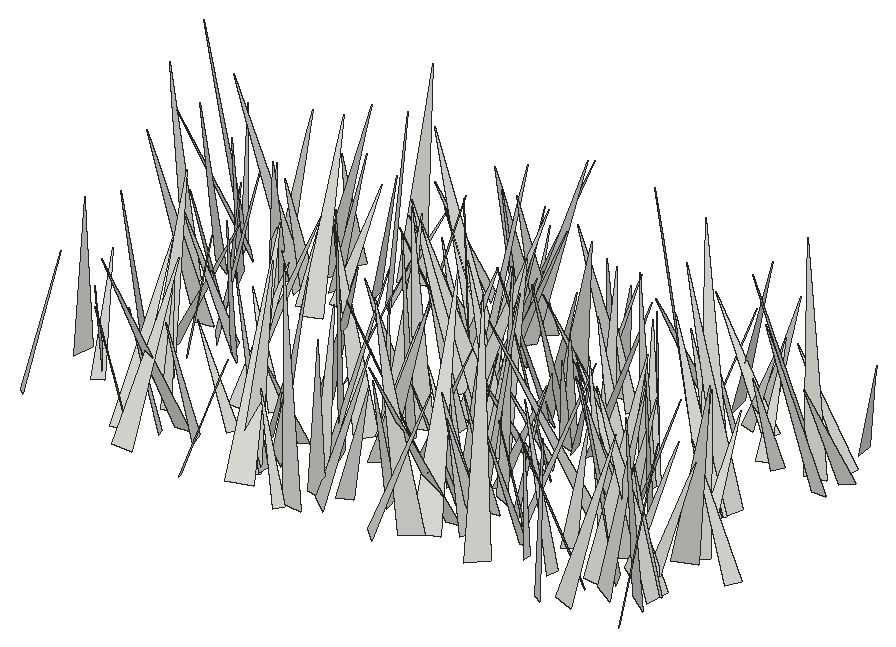
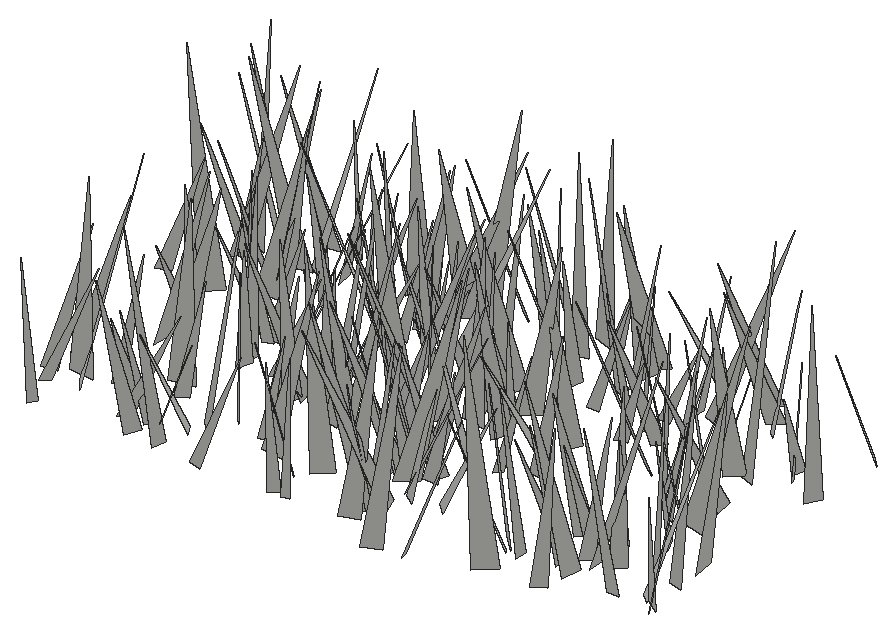
# SketchUp Ruby script. Lengths in inches.
U = 1.inch
M = Sketchup.active_model
def pt(a) = Geom::Point3d.new(a.map { |v| v * U })
def face(e, loops, mat)
  f = e.add_face(loops[0].map { |a| pt(a) })
  loops[1..].each { |l| e.add_face(l.map { |a| pt(a) }).erase! }
  f.material = f.back_material = mat if mat
  f
end
# faces: each face lists its corners as indices into pts; further lists are holes
def faces(e, pts, list, mat = nil) = list.each { |f| face(e, (f[0].is_a?(Array) ? f : [f]).map { |l| l.map { |i| pts[i] } }, mat) }
# xy, xz, yz: faces in a plane at the given z, y or x. An outline is a flat list of corners, or four numbers for a rectangle; further outlines are holes
def ring(l) = l.size == 4 ? [[l[0], l[1]], [l[2], l[1]], [l[2], l[3]], [l[0], l[3]]] : l.each_slice(2).to_a
def flat(e, list, mat, &to3) = list.each { |f| face(e, (f[0].is_a?(Array) ? f : [f]).map { |l| ring(l).map { |u, v| to3.(u, v) } }, mat) }
def xy(e, z, list, mat = nil) = flat(e, list, mat) { |x, y| [x, y, z] }
def xz(e, y, list, mat = nil) = flat(e, list, mat) { |x, z| [x, y, z] }
def yz(e, x, list, mat = nil) = flat(e, list, mat) { |y, z| [x, y, z] }
def lines(e, pts, list) = list.each { |a, b| e.add_line(pt(pts[a]), pt(pts[b])) }
# prism: a flat outline (further loops are holes) pulled along v
def prism(e, loops, v, mat = nil)
  f = face(e, loops, mat); d = Geom::Vector3d.new(v.map { |x| x * U })
  f.pushpull(f.normal.samedirection?(d) ? d.length : -d.length)
end
def box(e, o, s, mat = nil) = prism(e, [[o, [o[0] + s[0], o[1], o[2]], [o[0] + s[0], o[1] + s[1], o[2]], [o[0], o[1] + s[1], o[2]]]], [0, 0, s[2]], mat)
def at(x, y, z, deg = 0) = Geom::Transformation.translation(pt([x, y, z])) * Geom::Transformation.rotation(ORIGIN, Z_AXIS, deg.degrees)
def axes(o, x, y, z) = Geom::Transformation.new([*x, 0, *y, 0, *z, 0, *pt(o).to_a, 1])
def part(name) = M.definitions.add(name)
# library, detail: a bought-in or finely detailed component or shape, given as its bounding box
def library(name, o, s) = part(name).tap { |d| box(d.entities, o, s) }
def detail(e, o, s) = box(e.add_group.entities, o, s)
def put(e, d, t, mat = nil) = e.add_instance(d, t).tap { |i| i.material = mat if mat }
def group(e, t, mat = nil) = e.add_group.tap { |g| g.transformation = t; g.material = mat if mat }.entities
root = M.entities
c1 = part("fur_instance\#9")
p = [[0.8125,0,1.79],[0.67,-0.02,1.48],[0,-0.11,0],[0,0.11,0]]
faces(c1.entities,p,[[0,1,2,3]])
put(root,c1,axes([469.1875,380.91,-21.66],[3.38601,2.0667,0.33408],[1.88033,-3.28152,1.24252],[-0.92044,0.89903,3.76728]))
put(root,c1,axes([476.36,381.6,-21.66],[-0.98772,3.5916,0.11089],[3.35733,0.88143,1.35606],[-1.28071,-0.45933,3.46934]))
put(root,c1,axes([476.99,382.05,-21.66],[1.25442,7.48082,2.76942],[7.81491,-1.71475,1.09211],[-1.59984,-2.51056,7.50623]))
put(root,c1,axes([477.25,384.18,-21.66],[0.11264,-6.37998,1.60761],[-6.5012,0.13924,1.0081],[1.01142,1.60553,6.30084]))
put(root,c1,axes([462.07,384.52,-21.66],[-3.11173,-3.4795,0.92655],[-3.33661,3.24675,0.98692],[1.3537,0.0043,4.56244]))
put(root,c1,axes([482.78,382.4,-21.66],[3.70587,4.25797,0.60198],[4.28884,-3.60158,-0.92773],[0.31394,-1.06043,5.56805]))
put(root,c1,axes([495.72,382.58,-21.66],[2.53366,4.26731,1.78001],[4.34271,-2.89305,0.75426],[-1.5872,-1.10369,4.90515]))
put(root,c1,axes([496.5,385.9375,-21.66],[-4.09518,-5.32392,0.52178],[-5.17841,4.11019,1.29512],[1.34181,-0.38619,6.5907]))
put(root,c1,axes([465.73,385.54,-21.66],[-1.54524,-6.7658,0.51217],[-6.71547,1.44992,-1.10738],[-0.96994,0.74015,6.85109]))
put(root,c1,axes([464.27,381.45,-21.66],[-1.14169,6.19263,0.48775],[6.13199,1.20279,-0.91762],[0.99261,-0.30768,6.22978]))
put(root,c1,axes([478.04,383.45,-21.66],[3.54049,4.95211,1.34575],[5.12044,-3.30078,-1.32493],[0.33991,-1.85767,5.94164]))
put(root,c1,axes([467.2,385.05,-21.66],[-4.25466,-1.2014,1.34721],[-0.93808,4.41863,0.97784],[1.54219,-0.62673,4.31153]))
put(root,c1,axes([484.75,383.99,-21.66],[1.79805,-6.87497,3.712],[-7.43664,-2.674,-1.35027],[-2.39594,3.14033,6.97674]))
put(root,c1,axes([497.25,383.15,-21.66],[1.23681,5.98503,1.54047],[6.1022,-0.934,-1.27052],[0.97821,-1.7408,5.97797]))
put(root,c1,axes([478.81,384.96,-21.66],[3.21186,-3.52218,0.8528],[-3.62385,-3.13,0.72104],[-0.02677,1.11644,4.71189]))
put(root,c1,axes([464.93,384.375,-21.66],[-3.69691,-1.68274,0.52652],[-1.75981,3.59718,-0.85985],[0.10916,1.00233,3.96981]))
put(root,c1,axes([485.88,386.71,-21.66],[-1.10699,-6.38687,0.31821],[-6.26084,1.01671,-1.37367],[-1.30201,0.54128,6.33487]))
put(root,c1,axes([501.52,383.35,-21.66],[-4.45958,-2.36263,3.46386],[-3.3219,5.07642,-0.81428],[2.55838,2.47306,4.98064]))
put(root,c1,axes([500.88,385.89,-21.66],[-3.13728,-6.42445,2.27927],[-6.51063,3.56742,1.09378],[2.01998,1.52023,7.06539]))
put(root,c1,axes([455.16,383.0625,-21.66],[3.04107,3.48011,0.59696],[3.3547,-3.09349,0.94446],[-1.10161,0.1866,4.52408]))
put(root,c1,axes([472.42,383.6875,-21.66],[-5.70861,3.53079,2.01517],[3.32922,6.05385,-1.17592],[2.33318,0.00055,6.60847]))
put(root,c1,axes([481.35,386.33,-21.66],[4.6906,-0.13116,1.94102],[0.35682,-4.92253,-1.19491],[-1.91244,-1.24013,4.53774]))
put(root,c1,axes([487.46,386.14,-21.66],[3.16597,-2.82128,1.36449],[-2.73379,-3.43456,-0.75836],[-1.53229,0.2984,4.17228]))
put(root,c1,axes([487.93,386.76,-21.66],[2.45481,-4.16097,0.8917],[-4.06011,-2.59844,-0.9479],[-1.27449,0.26329,4.73722]))
put(root,c1,axes([472.73,384.6,-21.66],[-6.0397,-1.24718,1.08354],[-1.47294,5.92489,-1.39057],[0.74831,1.59618,6.00831]))
put(root,c1,axes([462.74,383.22,-21.66],[-1.71935,6.00909,0.23442],[5.94835,1.73522,-0.85232],[0.8839,0.01135,6.19184]))
put(root,c1,axes([472.59,382.47,-21.66],[-4.41357,6.91206,0.00056],[6.86097,4.38103,-0.99489],[0.83882,0.53496,8.14041]))
put(root,c1,axes([472.5,386.22,-21.66],[-2.78435,-5.66723,3.39056],[-5.97834,3.72634,1.319],[2.80584,2.3158,6.17497]))
put(root,c1,axes([486.87,387.5,-21.66],[-3.71631,2.59474,2.95715],[3.6126,3.86147,1.15179],[1.55775,-2.76492,4.38373]))
put(root,c1,axes([489.99,383.9,-21.66],[-7.18499,4.19207,1.05141],[4.04317,7.24035,-1.23823],[1.52698,0.55406,8.22584]))
put(root,c1,axes([498.52,385.55,-21.66],[3.30058,6.51639,2.13105],[6.85171,-3.21879,-0.76942],[-0.24255,-2.25268,7.26396]))
put(root,c1,axes([494.46,385.62,-21.66],[-5.51822,-0.21879,0.79161],[-0.32668,5.51842,-0.75206],[0.75352,0.79022,5.4711]))
put(root,c1,axes([501.37,387.21,-21.66],[-7.04891,1.70289,1.4017],[1.92518,7.04086,1.12767],[1.07622,-1.44158,7.16347]))
put(root,c1,axes([492.04,386.14,-21.66],[-3.53666,-0.44387,1.07965],[-0.6619,3.59984,-0.68824],[0.96154,0.84544,3.49732]))
put(root,c1,axes([490.95,387.22,-21.66],[-2.05485,-3.90462,0.97999],[-3.96047,1.76344,-1.27819],[-0.72186,1.43981,4.22312]))
put(root,c1,axes([486.05,387.56,-21.66],[-2.14589,-4.13922,0.79032],[-4.13009,1.88974,-1.31675],[-0.83673,1.28775,4.4726]))
put(root,c1,axes([457.51,388.1,-21.66],[3.15596,1.30372,1.61225],[1.82364,-3.14251,-1.02861],[-0.98659,-1.6383,3.25603]))
put(root,c1,axes([470.65,387.78,-21.66],[3.7872,-0.0255,0.26622],[0.02172,-3.73751,-0.66706],[-0.26655,-0.66693,3.72808]))
put(root,c1,axes([483.1,388.82,-21.66],[-4.92734,-5.46841,0.2776],[-5.45988,4.87887,-0.80338],[-0.41255,0.74316,7.31688]))
put(root,c1,axes([501.12,387.38,-21.66],[-0.94166,-4.10224,1.61468],[-4.38512,0.70145,-0.77524],[-0.45421,1.73259,4.13692]))
put(root,c1,axes([498.1,387.43,-21.66],[-6.28358,-3.49392,1.76213],[-3.72095,6.36668,-0.64478],[1.21124,1.43309,7.16066]))
put(root,c1,axes([472.57,388.79,-21.66],[0.53786,-3.60504,0.14249],[-3.55289,-0.5543,-0.6129],[-0.62738,0.04841,3.59304]))
put(root,c1,axes([485.4375,384.55,-21.66],[-4.43994,6.98412,0.3729],[6.94517,4.45476,-0.74146],[0.82561,0.08476,8.24265]))
put(root,c1,axes([468.29,387.21,-21.66],[-1.80359,3.13263,0.44398],[3.00697,1.53819,1.36218],[-0.98418,-1.04117,3.34825]))
put(root,c1,axes([497.26,386.28,-21.66],[0.16612,7.76506,1.97129],[7.95416,0.07536,-0.96713],[0.95574,-1.97685,7.70638]))
put(root,c1,axes([463.5,386.73,-21.66],[0.00503,4.167,0.7042],[4.17874,-0.11,0.62111],[-0.63075,-0.69557,4.12045]))
put(root,c1,axes([468.43,389.13,-21.66],[4.23217,0.79223,1.75299],[1.35483,-4.23497,-1.35698],[-1.36567,-1.74623,4.08626]))
put(root,c1,axes([459.77,389.8,-21.66],[-3.5221,-6.63629,1.77015],[-6.5539,3.84233,1.36448],[2.0543,0.8804,7.38808]))
put(root,c1,axes([489.56,389.01,-21.66],[-3.13954,-2.86345,1.03549],[-2.74612,3.30524,0.81394],[1.31545,0.06589,4.17056]))
put(root,c1,axes([500.37,387.43,-21.66],[0.61438,4.77457,1.24038],[4.786,-0.27399,-1.3159],[1.1955,-1.35681,4.63059]))
put(root,c1,axes([475.31,387.11,-21.66],[-4.49774,2.41965,1.22715],[2.26445,4.65664,-0.88215],[1.49428,0.22634,5.03052]))
put(root,c1,axes([454.97,389.32,-21.66],[5.79339,-2.08626,1.56673],[-1.97661,-6.00002,-0.68061],[-1.70297,-0.13319,6.11985]))
put(root,c1,axes([496.99,390.07,-21.66],[1.49882,-6.76146,1.59023],[-6.75855,-1.79498,-1.262],[-1.60255,1.24632,6.80963]))
put(root,c1,axes([487.15,389.16,-21.66],[-0.77658,-4.10323,1.17838],[-4.23531,0.59015,-0.73621],[-0.53592,1.28194,4.11067]))
put(root,c1,axes([457.85,387.13,-21.66],[-3.33951,2.40161,0.05247],[2.31618,3.24301,-1.02031],[0.63702,0.79874,3.98485]))
put(root,c1,axes([497.44,387.4375,-21.66],[-6.80477,1.06742,0.77743],[0.9228,6.76292,-1.20833],[0.94457,1.0827,6.78117]))
put(root,c1,axes([493.25,388.74,-21.66],[3.51253,-2.51047,1.78394],[-2.89575,-3.6135,0.61652],[-1.0486,1.56939,4.2732]))
put(root,c1,axes([482.89,390.39,-21.66],[3.48904,-1.79502,0.75996],[-1.60226,-3.52839,-0.97792],[-1.11014,-0.54905,3.7999]))
put(root,c1,axes([488.62,389.24,-21.66],[2.69077,3.3772,1.27263],[3.60609,-2.57991,-0.77814],[-0.14558,-1.48455,4.24737]))
put(root,c1,axes([498.06,388.5,-21.66],[2.30047,4.4169,0.81433],[4.47004,-2.16262,-0.89782],[0.43686,-1.13065,4.89848]))
put(root,c1,axes([487.16,387.67,-21.66],[4.31579,6.0344,1.65644],[5.97789,-4.5707,1.07586],[-1.85004,-0.69181,7.34048]))
put(root,c1,axes([475.23,387.58,-21.66],[4.30738,5.01035,0.65824],[4.94004,-4.35705,0.83813],[-1.06435,0.05398,6.55397]))
put(root,c1,axes([477.54,389.88,-21.66],[5.60342,-3.67276,1.04707],[-3.81273,-5.48708,1.15708],[-0.22057,1.54484,6.59914]))
put(root,c1,axes([489.59,388.76,-21.66],[4.90909,4.36789,0.50992],[4.39704,-4.86378,-0.66882],[0.06695,-0.83837,6.53684]))
put(root,c1,axes([475.34,389.01,-21.66],[-6.98093,-2.98191,2.95578],[-3.56155,7.24267,-1.10492],[2.22346,2.23913,7.51028]))
put(root,c1,axes([485.04,388.72,-21.66],[-4.58169,-0.00231,0.33908],[-0.10273,4.38765,-1.35823],[0.32316,1.36211,4.37574]))
put(root,c1,axes([483.6,390.89,-21.66],[0.23103,-4.99246,1.62863],[-5.17408,0.0623,0.92493],[0.89778,1.64376,4.91147]))
put(root,c1,axes([499.92,391.71,-21.66],[4.60789,-6.31495,1.14074],[-6.41656,-4.51508,0.92427],[0.08686,1.46561,7.76253]))
put(root,c1,axes([483.45,390.375,-21.66],[-2.38468,3.13652,0.12042],[3.02513,2.25628,1.13874],[-0.83714,-0.7813,3.77197]))
put(root,c1,axes([491.6,393.03,-21.66],[-6.74137,-3.47517,0.05647],[-3.44773,6.70195,0.85032],[0.43951,-0.73012,7.53656]))
put(root,c1,axes([484.39,389.58,-21.66],[3.67967,2.76321,1.03507],[2.46473,-3.78797,1.35021],[-1.62229,0.51247,4.39911]))
put(root,c1,axes([466.65,389.73,-21.66],[-1.32926,4.80497,0.97182],[4.66035,1.55098,-1.29408],[1.52094,-0.553,4.81456]))
put(root,c1,axes([460.62,389.86,-21.66],[-3.43213,5.64571,1.59286],[5.69776,3.64732,-0.65059],[1.39526,-1.00684,6.57497]))
put(root,c1,axes([468.8125,390.79,-21.66],[-2.26305,3.25436,0.20739],[3.19812,2.16563,0.91504],[-0.63708,-0.68879,3.8568]))
put(root,c1,axes([503.85,391.49,-21.66],[-3.48001,3.233,0.8636],[3.33945,3.27515,1.19585],[-0.21495,-1.45934,4.59703]))
put(root,c1,axes([486.45,390.75,-21.66],[3.17531,6.56755,2.54139],[6.79761,-3.58673,0.77578],[-1.83954,-1.91744,7.25351]))
put(root,c1,axes([470.55,393.24,-21.66],[6.6655,-1.52718,0.22941],[-1.49066,-6.62814,-0.81212],[-0.40351,-0.74118,6.78982]))
put(root,c1,axes([485.29,391.79,-21.66],[4.11337,-1.35782,0.42666],[-1.42017,-4.00175,0.95638],[-0.09392,1.04301,4.22479]))
put(root,c1,axes([475.1,391.68,-21.66],[-5.2406,4.407,1.34408],[4.57378,5.22157,0.71269],[0.55566,-1.41624,6.81011]))
put(root,c1,axes([479.43,391.75,-21.66],[4.44559,-0.41699,0.42413],[-0.48383,-4.39553,0.74982],[-0.34594,0.78895,4.4017]))
put(root,c1,axes([459.94,393.31,-21.66],[4.41125,2.39111,1.26664],[2.67652,-4.21168,-1.37073],[-0.39751,-1.82353,4.82677]))
put(root,c1,axes([475.95,391.98,-21.66],[1.17442,4.10835,0.87727],[4.16659,-1.02282,-0.78793],[0.5364,-1.0501,4.19964]))
put(root,c1,axes([493.22,394.3125,-21.66],[1.75124,-3.26229,0.83742],[-3.12175,-1.92651,-0.97669],[-1.26432,0.23809,3.57148]))
put(root,c1,axes([486.37,394.67,-21.66],[-0.29394,-4.28793,0.2812],[-4.0742,0.18848,-1.38464],[-1.36614,0.36048,4.06885]))
put(root,c1,axes([486.57,395.07,-21.66],[-3.34858,-4.98605,1.16696],[-4.83329,3.53804,1.24784],[1.69169,0.23891,5.87509]))
put(root,c1,axes([462.59,394.46,-21.66],[-2.53313,-4.37285,1.78451],[-4.47538,2.86942,0.67851],[1.50904,1.16947,5.00781]))
put(root,c1,axes([475.53,393.1,-21.66],[-3.90689,0.46662,1.17538],[0.26281,4.03296,-0.72751],[1.23701,0.61693,3.86682]))
put(root,c1,axes([465.07,392.66,-21.66],[3.93505,4.96293,0.50565],[4.97977,-3.8695,-0.7745],[0.29702,-0.87596,6.28613]))
put(root,c1,axes([462.05,395.3,-21.66],[-5.06877,-1.96642,0.89661],[-1.81084,5.11214,0.97466],[1.17965,-0.60192,5.34876]))
put(root,c1,axes([477.48,393.1,-21.66],[-6.31895,-1.30533,1.91515],[-1.71826,6.37081,-1.32708],[1.5554,1.73484,6.31441]))
put(root,c1,axes([500.5,392.71,-21.66],[-4.9436,1.78617,0.77223],[1.56135,4.89918,-1.33648],[1.16143,1.01666,5.08364]))
put(root,c1,axes([460.6,396.43,-21.66],[-3.28751,-5.48957,1.02333],[-5.33666,3.43821,1.29963],[1.64396,0.18343,6.2653]))
put(root,c1,axes([494.35,395.26,-21.66],[-4.3896,-2.50757,2.34029],[-2.3133,4.97071,0.98703],[2.5325,0.19407,4.95805]))
put(root,c1,axes([458.72,393.37,-21.66],[4.92318,-0.35306,0.35659],[-0.43613,-4.74982,1.31852],[-0.24819,1.34315,4.75646]))
put(root,c1,axes([493.17,394.65,-21.66],[0.04539,-4.24616,1.86431],[-4.44886,0.48634,1.21602],[1.30888,1.80033,4.06857]))
put(root,c1,axes([482.85,394.65,-21.66],[-2.73382,6.12597,3.74599],[6.6709,3.64992,-1.10045],[2.6569,-2.86083,6.61742]))
put(root,c1,axes([486.19,396.1,-21.66],[-3.41179,-1.77285,0.16017],[-1.67154,3.30984,1.02951],[0.61205,-0.84317,3.70451]))
put(root,c1,axes([479.12,395.76,-21.66],[-5.12264,0.34016,1.65759],[0.60899,5.30124,0.79415],[1.57874,-0.94118,5.07212]))
put(root,c1,axes([494.16,393.77,-21.66],[3.89284,1.77366,0.49192],[1.64576,-3.86945,0.92782],[-0.82421,0.65077,4.17603]))
put(root,c1,axes([458.6,396.52,-21.66],[-0.74223,-7.02206,1.66779],[-7.14663,0.48084,-1.156],[-1.00829,1.76103,6.96591]))
put(root,c1,axes([477.17,394.66,-21.66],[-0.74799,6.94474,2.29097],[7.27165,0.46217,0.97314],[-0.77532,-2.36525,6.91678]))
put(root,c1,axes([481.41,396.45,-21.66],[-7.37091,1.53228,0.84327],[1.65266,7.29739,1.18581],[0.57246,-1.33774,7.43452]))
put(root,c1,axes([460.25,395.67,-21.66],[4.87544,3.99495,1.42226],[4.19795,-4.85335,-0.75795],[-0.59966,-1.4959,6.2574]))
put(root,c1,axes([474.77,394.83,-21.66],[-5.03968,3.97301,2.20808],[3.85689,5.48236,-1.06156],[2.40517,-0.46656,6.329]))
put(root,c1,axes([485.34,398.3125,-21.66],[-0.07367,-4.26522,0.50041],[-4.16979,0.19077,1.01214],[1.02732,0.46845,4.14405]))
put(root,c1,axes([469.96,397.4,-21.66],[-0.83956,4.61048,2.28414],[5.1209,0.52371,0.82514],[-0.50027,-2.37653,4.61309]))
put(root,c1,axes([498.55,395.55,-21.66],[-1.96871,3.37657,0.07437],[3.27614,1.93014,-0.90775],[0.82077,0.39482,3.80171]))
put(root,c1,axes([490.25,397.57,-21.66],[-3.73947,1.85603,0.44676],[1.90802,3.6015,1.00834],[-0.06253,-1.10111,4.05114]))
put(root,c1,axes([485.99,398.41,-21.66],[4.14097,0.37336,0.37849],[0.46882,-3.96604,-1.21698],[-0.25072,-1.24957,3.97567]))
put(root,c1,axes([472.2,398.46,-21.66],[-3.76395,0.54517,1.33918],[0.93594,3.7652,1.09781],[1.1021,-1.33566,3.64133]))
put(root,c1,axes([485.17,398.96,-21.66],[0.2797,-5.08952,0.70223],[-5.01624,-0.11848,1.13926],[1.11073,0.74654,4.96825]))
put(root,c1,axes([497.95,397.1,-21.66],[-4.76226,4.46867,0.77555],[4.53262,4.64929,1.04363],[-0.16086,-1.29026,6.44663]))
put(root,c1,axes([492.59,397.24,-21.66],[-6.8831,0.44539,2.18741],[0.27023,7.20464,-0.61666],[2.21588,0.50489,6.86987]))
put(root,c1,axes([482.55,400.25,-21.66],[-2.90954,-6.16313,0.64564],[-6.10361,2.97343,0.8781],[1.07095,0.20243,6.75859]))
put(root,c1,axes([469.79,396.34,-21.66],[4.40688,2.08061,0.00975],[2.02682,-4.29803,1.08102],[-0.47012,0.97349,4.75194]))
put(root,c1,axes([488.1,400.23,-21.66],[-5.70608,-2.81682,0.48614],[-2.67601,5.6456,1.30244],[1.0049,-0.96065,6.22877]))
put(root,c1,axes([483.9,400.15,-21.66],[-1.823,-5.96341,0.88128],[-5.94354,1.93183,0.77754],[1.00658,0.60664,6.18716]))
put(root,c1,axes([482.34,399.99,-21.66],[6.03259,-1.06555,0.38284],[-1.02373,-6.01977,-0.62323],[-0.48366,-0.54868,6.09418]))
put(root,c1,axes([492.49,397.8,-21.66],[-4.5808,2.50643,0.71678],[2.42315,4.62824,-0.69815],[0.96142,0.27723,5.1748]))
put(root,c1,axes([478.18,397.43,-21.66],[3.15625,6.97995,0.87784],[7.00121,-3.02246,-1.14023],[0.68808,-1.26383,7.57506]))
put(root,c1,axes([498.39,398.24,-21.66],[-7.87651,1.28049,0.44694],[1.23259,7.85729,-0.78901],[0.56579,0.70864,7.94081]))
put(root,c1,axes([476.51,400.09,-21.66],[-4.90081,-4.60842,2.76686],[-4.75517,5.4628,0.67611],[2.50627,1.35324,6.69315]))
put(root,c1,axes([488.52,399.6,-21.66],[-2.55012,3.64542,1.48438],[3.93085,2.44958,0.73729],[0.20222,-1.64502,4.38733]))
put(root,c1,axes([487.19,398.43,-21.66],[5.64038,0.84844,0.8162],[0.68974,-5.61874,1.07421],[-0.95409,0.95384,5.60177]))
put(root,c1,axes([478.86,399.54,-21.66],[-2.03282,4.17049,1.29504],[4.34211,1.77825,1.08919],[-0.46493,-1.62705,4.50988]))
put(root,c1,axes([476.25,399.84,-21.66],[-6.01632,2.22797,0.81671],[2.32649,5.97644,0.83455],[0.46722,-1.07014,6.36109]))
put(root,c1,axes([458.35,399.03,-21.66],[-3.5127,-1.06556,1.8883],[-1.54789,3.74984,-0.76344],[1.51826,1.35772,3.59049]))
put(root,c1,axes([487.5,399.42,-21.66],[4.97353,-2.18793,2.98402],[-2.79783,-5.49524,0.634],[-2.42149,1.85546,5.39639]))
put(root,c1,axes([454.93,400.0625,-21.66],[-7.05246,-0.20222,1.59365],[-0.38202,7.18084,-0.77939],[1.56034,0.84409,7.01218]))
put(root,c1,axes([454.98,402.74,-21.66],[-2.48382,-6.27006,1.58629],[-6.2632,2.75568,1.08533],[1.61318,1.04494,6.65621]))
put(root,c1,axes([476.97,401.16,-21.66],[3.46953,-2.67132,1.40146],[-2.94376,-3.4648,0.68347],[-0.65905,1.41311,4.3251]))
put(root,c1,axes([474.43,401.2,-21.66],[3.70527,-2.55389,0.75103],[-2.66189,-3.54115,1.0909],[0.02774,1.32414,4.36593]))
put(root,c1,axes([456.74,402.43,-21.66],[4.97052,1.68586,2.30908],[2.28367,-5.12743,-1.17229],[-1.72012,-1.9358,5.11604]))
put(root,c1,axes([460.83,400.44,-21.66],[0.97276,4.45119,0.9772],[4.35496,-1.20232,1.14148],[-1.3425,-0.67498,4.41093]))
put(root,c1,axes([459.04,403.24,-21.66],[4.90376,-2.85552,0.72078],[-2.73926,-4.93651,-0.92072],[-1.08166,-0.44414,5.59939]))
put(root,c1,axes([475.1,403.62,-21.66],[-5.50457,-1.9976,0.13924],[-1.94432,5.42927,1.02602],[0.47897,-0.91798,5.76524]))
put(root,c1,axes([474.72,401.92,-21.66],[0.57769,-3.84784,2.16026],[-4.16363,-1.197,-1.01866],[-1.46176,1.88882,3.75525]))
put(root,c1,axes([461.22,403.5625,-21.66],[3.60801,-2.69307,1.35493],[-2.4926,-3.85347,-1.02171],[-1.69571,-0.06573,4.3848]))
put(root,c1,axes([470.25,402.59,-21.66],[6.04949,2.12455,0.78775],[2.22415,-5.99674,-0.90711],[-0.43293,-1.1207,6.34722]))
put(root,c1,axes([500.96,403.39,-21.66],[-1.48365,-5.76059,1.44193],[-5.8771,1.21156,-1.20691],[-0.85046,1.67706,5.82486]))
put(root,c1,axes([455.41,405.1,-21.66],[-4.43936,-4.76816,0.23664],[-4.66276,4.39992,1.18262],[1.02469,-0.63608,6.40661]))
put(root,c1,axes([488.52,403.39,-21.66],[3.47548,2.68418,2.07766],[3.24177,-3.50628,-0.89294],[-1.00618,-2.02524,4.29959]))
put(root,c1,axes([460.34,403.73,-21.66],[-7.46338,-1.41905,1.28497],[-1.31215,7.55774,0.72509],[1.39396,-0.48353,7.56241]))
put(root,c1,axes([475.88,402.72,-21.66],[-6.89397,4.20656,1.53795],[4.42912,6.82252,1.19307],[0.66584,-1.82904,7.9874]))
put(root,c1,axes([477.26,401.9,-21.66],[6.02676,-0.13267,0.65935],[-0.25057,-5.95995,1.09109],[-0.62414,1.1116,5.92866]))
put(root,c1,axes([474.29,404.48,-21.66],[-3.67064,-4.64361,1.03864],[-4.58105,3.8034,0.81465],[1.28682,0.29416,5.86285]))
put(root,c1,axes([497.07,404.31,-21.66],[2.57242,-3.23839,0.522],[-3.12857,-2.6216,-0.84629],[-0.98573,-0.13048,4.04824]))
put(root,c1,axes([493.08,403.17,-21.66],[-3.28307,2.60382,1.30489],[2.8552,3.26547,0.66758],[0.57484,-1.34832,4.13676]))
put(root,c1,axes([462.01,401.91,-21.66],[-2.71251,3.20119,0.88639],[3.03008,2.85354,-1.03292],[1.36084,0.02704,4.06674]))
put(root,c1,axes([494.09,401.875,-21.66],[-3.06885,7.2619,1.47031],[7.40414,2.94663,0.90053],[-0.27521,-1.70206,7.83212]))
put(root,c1,axes([480.46,405.19,-21.66],[3.94338,-5.9757,0.15667],[-5.94055,-3.89659,0.90015],[0.66588,0.62564,7.10275]))
put(root,c1,axes([463.16,401.3,-21.66],[-3.56616,5.34471,0.77163],[5.27091,3.64619,-0.89538],[1.17426,-0.13507,6.36253]))
put(root,c1,axes([501.57,405.45,-21.66],[1.96703,-4.29578,0.10046],[-4.18734,-1.94112,-1.01553],[-0.96439,-0.33368,4.61429]))
put(root,c1,axes([472.08,404.16,-21.66],[-2.77092,-3.22119,0.17285],[-3.17409,2.68192,-0.90354],[-0.57541,0.71776,4.15182]))
put(root,c1,axes([476.3,401.1875,-21.66],[3.93079,5.90323,1.06815],[5.73682,-4.07234,1.39466],[-1.7544,-0.09002,6.95371]))
put(root,c1,axes([477.33,402.125,-21.66],[-3.93965,-2.75758,3.63418],[-3.8658,4.56754,-0.72493],[2.42222,2.80458,4.7539]))
put(root,c1,axes([498.85,405.86,-21.66],[-5.87389,-5.06073,1.31002],[-4.91563,6.01764,1.20596],[1.77871,-0.08191,7.65893]))
put(root,c1,axes([485.84,404.15,-21.66],[1.13242,-3.28388,1.61058],[-3.44754,-1.52145,-0.67814],[-1.2216,1.24962,3.40681]))
put(root,c1,axes([484.38,405.24,-21.66],[0.42808,-6.23217,1.75974],[-6.34467,-0.7568,-1.13683],[-1.29687,1.64535,6.14254]))
put(root,c1,axes([463.53,403.24,-21.66],[-0.65991,4.20046,0.70673],[4.09857,0.8209,-1.05196],[1.15975,-0.51096,4.1198]))
put(root,c1,axes([464.65,405.67,-21.66],[5.2345,0.58731,0.96902],[0.7581,-5.21929,-0.93179],[-0.84215,-1.04786,5.18428]))
put(root,c1,axes([476.94,404.77,-21.66],[-3.42512,-4.29344,1.99666],[-4.721,3.28594,-1.03273],[0.36395,2.21827,5.39431]))
put(root,c1,axes([462.21,404.72,-21.66],[4.7492,-0.22527,1.39473],[-0.44396,-4.88167,0.72329],[-1.34124,0.81823,4.6992]))
put(root,c1,axes([489.3,405.5,-21.66],[-5.53788,-5.2946,2.37412],[-5.70348,5.57065,-0.88067],[1.06751,2.29618,7.61087]))
put(root,c1,axes([454.62,405.59,-21.66],[-6.58446,-3.61184,1.85584],[-3.84727,6.67992,-0.64953],[1.29924,1.4758,7.48189]))
put(root,c1,axes([499.61,404.8,-21.66],[-0.81741,7.52572,2.31704],[7.8363,0.54876,0.98214],[-0.77303,-2.39493,7.506]))
put(root,c1,axes([465.74,405.8,-21.66],[3.62695,2.69385,0.06353],[2.59465,-3.4627,-1.30122],[0.7271,-1.08099,4.32648]))
put(root,c1,axes([460.81,405.55,-21.66],[6.40804,-1.16691,1.44574],[-1.35043,-6.49108,0.74636],[-1.27601,1.00946,6.47052]))
put(root,c1,axes([457.27,405.92,-21.66],[1.6675,5.06938,1.93589],[5.41393,-1.41673,-0.95346],[0.36831,-2.12629,5.25072]))
put(root,c1,axes([495.77,404.45,-21.66],[-2.69846,2.82224,0.09608],[2.72603,2.63813,-0.93001],[0.73688,0.57546,3.79233]))
put(root,c1,axes([500.89,406.68,-21.66],[-4.33776,1.46199,0.55548],[1.55819,4.18055,1.16497],[0.13425,-1.28363,4.42678]))
put(root,c1,axes([466.2,404.9,-21.66],[3.82909,4.88275,1.88302],[4.81565,-4.20088,1.10051],[-2.04855,-0.74856,6.10673]))
put(root,c1,axes([475.77,408.5,-21.66],[3.11864,-5.68803,0.55795],[-5.6529,-3.16353,-0.65398],[-0.84244,0.17118,6.45383]))
put(root,c1,axes([454.52,405.58,-21.66],[1.72426,4.07776,1.35625],[4.04188,-2.03524,0.98061],[-1.4597,-0.81871,4.31736]))
put(root,c1,axes([492.26,406.11,-21.66],[-3.43885,-1.25141,0.28396],[-1.28081,3.29756,-0.97876],[-0.07859,1.01608,3.52615]))
put(root,c1,axes([481.72,406.48,-21.66],[3.27603,2.91205,0.73309],[2.99826,-3.11162,-1.03833],[0.1671,-1.26001,4.25844]))
put(root,c1,axes([461.38,408.03,-21.66],[3.51488,-3.51732,0.75482],[-3.443,-3.59499,-0.71937],[-1.04262,0.01399,4.9202]))
put(root,c1,axes([492.47,407.07,-21.66],[0.8957,-3.44027,0.95903],[-3.38159,-0.49886,1.36875],[1.14894,1.21373,3.28089]))
put(root,c1,axes([494.3,407.21,-21.66],[-4.30239,2.31555,0.00735],[2.25428,4.18495,1.12996],[-0.52922,-0.99839,4.75348]))
put(root,c1,axes([475.25,407.25,-21.66],[1.48907,3.83094,1.46531],[4.09712,-1.31638,-0.722],[0.19182,-1.62223,4.04625]))
put(root,c1,axes([475.52,406.74,-21.66],[6.84778,-1.68967,1.39359],[-1.92956,-6.81846,1.21431],[-1.03628,1.53061,6.94784]))
put(root,c1,axes([490.17,406.11,-21.66],[3.37937,2.22818,0.23171],[2.15143,-3.34494,0.78826],[-0.62436,0.53406,3.97033]))
put(root,c1,axes([490.44,408.6875,-21.66],[6.84395,0.46131,0.76105],[0.6015,-6.74756,-1.31919],[-0.65589,-1.3745,6.73144]))
put(root,c1,axes([481.35,408.85,-21.66],[1.83451,-3.56347,0.05806],[-3.52397,-1.80394,0.62811],[0.53227,0.33851,3.95843]))
put(root,c1,axes([480.33,408.99,-21.66],[-0.97115,-4.17934,0.95629],[-4.09852,1.19278,1.05068],[1.25838,0.65947,4.16006]))
put(root,c1,axes([474.66,406.07,-21.66],[6.67299,1.88656,0.54903],[1.75109,-6.59185,1.3677],[-0.89119,1.17381,6.79833]))
put(root,c1,axes([487.18,409.28,-21.66],[-0.13278,-3.81265,0.23397],[-3.74221,0.08288,-0.77308],[-0.76609,0.25594,3.73581]))
put(root,c1,axes([499.81,409.28,-21.66],[4.41728,-0.60705,0.29796],[-0.51929,-4.30631,-1.07505],[-0.43316,-1.02804,4.32726]))
put(root,c1,axes([465.32,408.35,-21.66],[-3.47226,6.33449,3.63746],[6.89094,4.17667,-0.69553],[2.42317,-2.80055,7.19017]))
put(root,c1,axes([492.625,408.5,-21.66],[4.10289,-2.86128,0.97197],[-3.01034,-4.01302,0.89377],[-0.2636,1.29386,4.92156]))
put(root,c1,axes([472.33,410.63,-21.66],[3.11347,-5.57932,0.56956],[-5.54553,-3.1599,-0.63956],[-0.83685,0.18197,6.35716]))
put(root,c1,axes([470.2,410.15,-21.66],[-4.41173,-1.92667,0.46008],[-1.77307,4.34177,1.17998],[0.88316,-0.90777,4.66723]))
